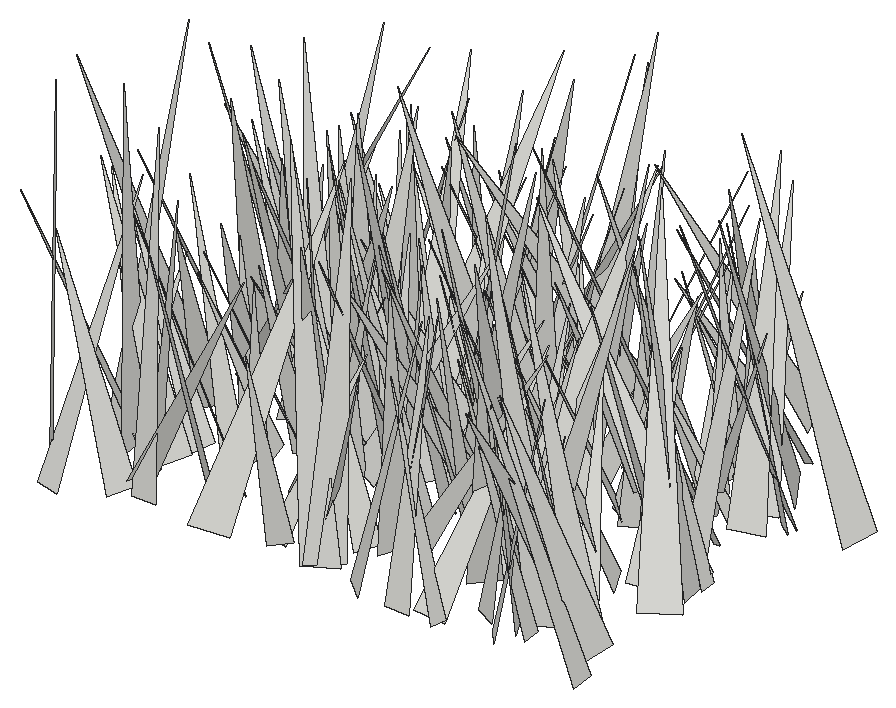
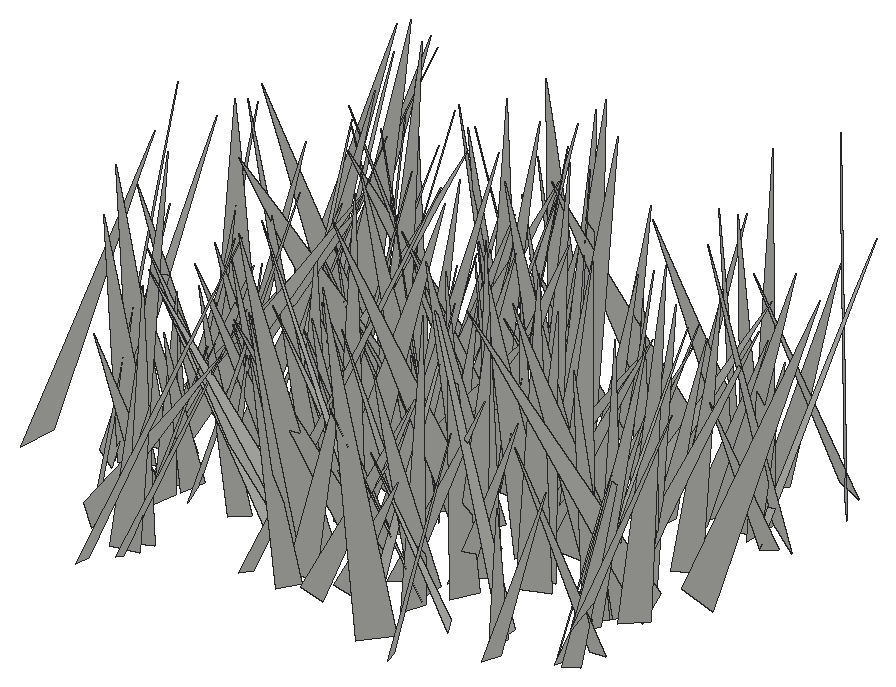
# SketchUp Ruby script. Lengths in inches.
U = 1.inch
M = Sketchup.active_model
def pt(a) = Geom::Point3d.new(a.map { |v| v * U })
def face(e, loops, mat)
  f = e.add_face(loops[0].map { |a| pt(a) })
  loops[1..].each { |l| e.add_face(l.map { |a| pt(a) }).erase! }
  f.material = f.back_material = mat if mat
  f
end
# faces: each face lists its corners as indices into pts; further lists are holes
def faces(e, pts, list, mat = nil) = list.each { |f| face(e, (f[0].is_a?(Array) ? f : [f]).map { |l| l.map { |i| pts[i] } }, mat) }
# xy, xz, yz: faces in a plane at the given z, y or x. An outline is a flat list of corners, or four numbers for a rectangle; further outlines are holes
def ring(l) = l.size == 4 ? [[l[0], l[1]], [l[2], l[1]], [l[2], l[3]], [l[0], l[3]]] : l.each_slice(2).to_a
def flat(e, list, mat, &to3) = list.each { |f| face(e, (f[0].is_a?(Array) ? f : [f]).map { |l| ring(l).map { |u, v| to3.(u, v) } }, mat) }
def xy(e, z, list, mat = nil) = flat(e, list, mat) { |x, y| [x, y, z] }
def xz(e, y, list, mat = nil) = flat(e, list, mat) { |x, z| [x, y, z] }
def yz(e, x, list, mat = nil) = flat(e, list, mat) { |y, z| [x, y, z] }
def lines(e, pts, list) = list.each { |a, b| e.add_line(pt(pts[a]), pt(pts[b])) }
# prism: a flat outline (further loops are holes) pulled along v
def prism(e, loops, v, mat = nil)
  f = face(e, loops, mat); d = Geom::Vector3d.new(v.map { |x| x * U })
  f.pushpull(f.normal.samedirection?(d) ? d.length : -d.length)
end
def box(e, o, s, mat = nil) = prism(e, [[o, [o[0] + s[0], o[1], o[2]], [o[0] + s[0], o[1] + s[1], o[2]], [o[0], o[1] + s[1], o[2]]]], [0, 0, s[2]], mat)
def at(x, y, z, deg = 0) = Geom::Transformation.translation(pt([x, y, z])) * Geom::Transformation.rotation(ORIGIN, Z_AXIS, deg.degrees)
def axes(o, x, y, z) = Geom::Transformation.new([*x, 0, *y, 0, *z, 0, *pt(o).to_a, 1])
def part(name) = M.definitions.add(name)
# library, detail: a bought-in or finely detailed component or shape, given as its bounding box
def library(name, o, s) = part(name).tap { |d| box(d.entities, o, s) }
def detail(e, o, s) = box(e.add_group.entities, o, s)
def put(e, d, t, mat = nil) = e.add_instance(d, t).tap { |i| i.material = mat if mat }
def group(e, t, mat = nil) = e.add_group.tap { |g| g.transformation = t; g.material = mat if mat }.entities
root = M.entities
c1 = part("fur_instance\#9")
p = [[0.8125,0,1.79],[0.67,-0.02,1.48],[0,-0.11,0],[0,0.11,0]]
faces(c1.entities,p,[[0,1,2,3]])
put(root,c1,axes([74.77,271.22,-27.1],[2.46831,-3.73303,1.12427],[-3.72872,-2.64901,-0.60947],[-1.13849,0.58247,4.43358]))
put(root,c1,axes([89.13,272.08,-27.1],[5.01755,-2.86523,2.69296],[-2.1597,-5.65647,-1.99435],[-3.28592,-0.6574,5.42291]))
put(root,c1,axes([90.02,270.07,-27.1],[-7.1325,-1.97369,0.04131],[-1.9512,7.0246,-1.27181],[-0.29997,1.23662,7.29044]))
put(root,c1,axes([67.68,270.7,-27.1],[-4.78062,2.36193,1.12593],[2.54726,4.73726,0.87783],[0.59826,-1.2963,5.25951]))
put(root,c1,axes([64.64,270.28,-27.1],[-5.7343,-4.84539,3.53032],[-5.45543,6.24306,-0.29262],[2.4858,2.5238,7.50162]))
put(root,c1,axes([71.45,271.63,-27.1],[-3.14093,-4.54056,1.19879],[-4.68857,3.11384,-0.49041],[0.26658,1.26749,5.49924]))
put(root,c1,axes([83.08,270.24,-27.1],[-4.76571,-0.2474,0.30777],[-0.30187,4.68534,-0.90794],[0.25457,0.92426,4.68496]))
put(root,c1,axes([86.31,274.4,-27.1],[4.64507,-4.79979,0.2726],[-4.36308,-4.36804,-2.56373],[-2.01887,-1.6035,6.16782]))
put(root,c1,axes([76.08,272.24,-27.1],[5.21952,0.68023,0.61562],[0.83808,-4.98198,-1.60081],[-0.37326,-1.674,5.01433]))
put(root,c1,axes([79.03,270.31,-27.1],[3.65147,4.43575,1.22236],[4.5601,-3.69672,-0.20725],[-0.61278,-1.07778,5.74161]))
put(root,c1,axes([81.28,270,-27.1],[0.82489,5.68831,1.342],[5.81529,-0.93413,0.38496],[-0.58339,-1.2684,5.73491]))
put(root,c1,axes([85.58,271.84,-27.1],[3.95748,1.9361,2.48086],[2.44941,-4.39763,-0.47534],[-1.97573,-1.57388,4.37997]))
put(root,c1,axes([84.11,271.7,-27.1],[-0.58036,-3.55618,1.37675],[-3.59236,0.97706,1.00942],[1.27936,1.13031,3.45894]))
put(root,c1,axes([85.32,270.69,-27.1],[3.56693,3.32971,1.1246],[3.34181,-3.70943,0.38354],[-1.08812,-0.47732,4.86445]))
put(root,c1,axes([67.83,271.52,-27.1],[5.28703,-2.12696,0.17156],[-2.11759,-5.17319,1.12251],[0.26309,1.10465,5.58719]))
put(root,c1,axes([79.96,271.45,-27.1],[5.42096,2.25752,1.64956],[2.38588,-5.61122,-0.16143],[-1.45775,-0.7887,5.87002]))
put(root,c1,axes([65.36,269.17,-27.1],[2.05142,5.93925,0.09208],[5.90467,-2.04959,0.65232],[-0.64654,0.12643,6.2496]))
put(root,c1,axes([86.4,271.58,-27.1],[-5.31837,-1.43549,0.4315],[-1.49067,5.23198,-0.96754],[0.15722,1.04767,5.42306]))
put(root,c1,axes([65.6,274.26,-27.1],[-4.61159,-4.4726,0.38091],[-4.39573,4.61032,0.9157],[0.90928,-0.396,6.35865]))
put(root,c1,axes([77.02,271.06,-27.1],[-5.99811,4.4385,2.51735],[4.45899,6.44808,-0.74453],[2.48087,-0.8583,7.4245]))
put(root,c1,axes([77.01,270.8,-27.1],[-1.50956,7.97784,1.83345],[8.07703,1.14872,1.65178],[-1.3301,-2.07864,7.94961]))
put(root,c1,axes([82.47,273.74,-27.1],[4.37125,-4.19897,0.80164],[-4.19734,-4.43318,-0.33332],[-0.81017,0.31203,6.05212]))
put(root,c1,axes([78.4,273.55,-27.1],[5.51508,-3.1001,1.56666],[-3.03836,-5.73026,-0.64316],[-1.68328,0.18611,6.29389]))
put(root,c1,axes([68.75,270.68,-27.1],[1.63726,6.8228,1.57078],[6.72877,-1.9791,1.58281],[-1.9343,-1.10957,6.83563]))
put(root,c1,axes([74.47,271.41,-27.1],[0.4921,4.23207,0.57816],[4.10963,-0.31046,-1.22532],[1.16432,-0.69285,4.08059]))
put(root,c1,axes([82.51,270.41,-27.1],[-2.22642,5.28944,0.76409],[4.89566,2.35054,-2.00661],[2.14349,0.12554,5.37668]))
put(root,c1,axes([67.1,273.39,-27.1],[3.49606,4.56093,2.47636],[5.16488,-3.35013,-1.12142],[-0.50841,-2.67048,5.63622]))
put(root,c1,axes([86.95,273.62,-27.1],[-5.18557,-4.32883,1.54546],[-4.49087,5.26797,-0.31293],[0.97941,1.23577,6.74766]))
put(root,c1,axes([86.36,272.54,-27.1],[-0.9931,7.68396,2.84346],[8.04191,0.36629,1.81887],[-1.56723,-2.98953,7.53135]))
put(root,c1,axes([77.51,273,-27.1],[-4.02277,2.62654,1.01722],[2.78428,3.97624,0.74391],[0.42575,-1.18612,4.74637]))
put(root,c1,axes([65.93,273.72,-27.1],[7.3985,0.06507,3.2704],[0.28828,-8.06925,-0.49163],[-3.25831,-0.56619,7.38244]))
put(root,c1,axes([72.08,270.36,-27.1],[-4.61251,5.93847,1.25396],[5.3205,4.71401,-2.75381],[2.92064,0.79104,6.99694]))
put(root,c1,axes([72.86,276.41,-27.1],[5.93446,-4.51627,0.11992],[-4.41947,-5.84426,-1.3935],[-0.93776,-1.03771,7.32616]))
put(root,c1,axes([71.45,273.29,-27.1],[-4.82792,-3.85999,0.34861],[-3.62589,4.30173,-2.58417],[-1.36894,2.21934,5.6152]))
put(root,c1,axes([67.8,273.71,-27.1],[-5.5849,2.54638,0.93821],[2.66389,5.55377,0.78405],[0.51763,-1.10771,6.08773]))
put(root,c1,axes([78.87,274.4375,-27.1],[4.45492,4.83666,0.95124],[4.56601,-3.56591,-3.25273],[1.85733,-2.83468,5.71483]))
put(root,c1,axes([87.88,273.12,-27.1],[-6.93734,1.12272,0.61983],[1.08478,6.95591,-0.45824],[0.68406,0.3553,7.01265]))
put(root,c1,axes([84.2,273.8125,-27.1],[-6.46812,-3.13785,1.21731],[-3.3431,6.29489,-1.53709],[0.38946,1.92167,7.02282]))
put(root,c1,axes([76.34,277.4,-27.1],[-2.99336,-6.46525,0.18966],[-6.30073,2.9619,1.52434],[1.46161,-0.47255,6.9596]))
put(root,c1,axes([74.34,274.375,-27.1],[-5.53367,-3.1899,2.46645],[-3.58117,5.81278,-0.51687],[1.85312,1.70777,6.3663]))
put(root,c1,axes([80.82,275.21,-27.1],[-3.26871,-2.2439,0.63682],[-2.29753,3.28654,-0.21245],[0.40248,0.53729,3.95909]))
put(root,c1,axes([74.2,274.79,-27.1],[-1.49797,-4.88201,2.75569],[-5.27998,2.18724,1.00478],[1.88406,2.24805,5.00683]))
put(root,c1,axes([70.18,275.58,-27.1],[3.44775,-2.42349,1.09947],[-2.43313,-3.5995,-0.30427],[-1.07797,0.37336,4.2033]))
put(root,c1,axes([80.49,275.58,-27.1],[-1.33118,-5.02308,1.66852],[-5.29255,1.28443,-0.35575],[0.06525,1.70478,5.18429]))
put(root,c1,axes([80.43,277.85,-27.1],[7.22069,-3.00234,1.05262],[-2.62839,-7.10035,-2.22196],[-1.79266,-1.6827,7.49769]))
put(root,c1,axes([86.3,276.83,-27.1],[-5.06216,-2.56794,0.53616],[-2.44101,5.03776,1.08155],[0.96086,-0.73072,5.57226]))
put(root,c1,axes([83.34,275.73,-27.1],[3.34183,1.38887,0.77255],[1.56239,-3.2005,-1.00466],[-0.29109,-1.23347,3.4767]))
put(root,c1,axes([67.99,275.08,-27.1],[-4.93751,1.50851,0.32737],[1.53378,4.91815,0.47027],[0.1741,-0.54591,5.14135]))
put(root,c1,axes([66.37,274.11,-27.1],[-3.43494,4.07646,0.13435],[4.04677,3.38429,0.77755],[-0.50915,-0.60283,5.27368]))
put(root,c1,axes([70.38,276.59,-27.1],[-4.26767,-0.91045,0.71231],[-0.70932,4.21373,1.13607],[0.91278,-0.98229,4.21323]))
put(root,c1,axes([79.55,277.92,-27.1],[1.60402,-6.13136,0.73735],[-5.58582,-1.76536,-2.52831],[-2.63361,0.00991,5.81155]))
put(root,c1,axes([78.98,274.86,-27.1],[-7.05105,-1.29004,0.36767],[-1.33665,6.92247,-1.34515],[0.11284,1.38992,7.04075]))
put(root,c1,axes([64.91,274.48,-27.1],[-0.81178,3.59213,0.55552],[3.51446,0.92094,-0.81938],[0.92765,-0.34562,3.5904]))
put(root,c1,axes([84.94,276,-27.1],[-4.9499,-5.12629,0.49866],[-4.98162,4.58947,-2.26921],[-1.30806,1.92014,6.75508]))
put(root,c1,axes([84.68,273.64,-27.1],[6.67924,-1.26552,2.75336],[-2.18749,-6.62541,2.26131],[-2.097,2.88046,6.41095]))
put(root,c1,axes([71.25,277.23,-27.1],[1.69834,-4.62751,0.65795],[-4.61755,-1.76962,-0.52709],[-0.72459,0.43091,4.90106]))
put(root,c1,axes([66.21,277.76,-27.1],[3.84252,-3.67557,0.42443],[-3.56655,-3.84235,-0.9854],[-0.98471,-0.42605,5.2253]))
put(root,c1,axes([75.875,276.62,-27.1],[-6.16765,-3.82155,1.90605],[-3.98751,6.35208,-0.16723],[1.52874,1.15063,7.2537]))
put(root,c1,axes([81.23,276.02,-27.1],[-3.53133,-2.30027,1.49102],[-2.55807,3.63918,-0.44418],[0.98523,1.20406,4.19097]))
put(root,c1,axes([71.56,276.83,-27.1],[-3.04212,-3.44962,0.11938],[-3.35963,2.92271,-1.15727],[-0.79185,0.85236,4.45141]))
put(root,c1,axes([65.06,273.51,-27.1],[3.59561,7.30217,1.1805],[7.09033,-3.77639,1.76345],[-2.10771,-0.24675,7.94609]))
put(root,c1,axes([72.86,276.56,-27.1],[1.59006,-7.38899,3.46765],[-7.94346,-2.21328,-1.07372],[-1.87702,3.10714,7.48148]))
put(root,c1,axes([69.16,275.47,-27.1],[-5.26641,1.25593,0.32091],[1.22212,5.2582,-0.5227],[0.43216,0.43524,5.3888]))
put(root,c1,axes([86.23,275.01,-27.1],[-2.52047,3.62206,0.22803],[3.61381,2.53037,-0.24846],[0.33426,-0.04477,4.40572]))
put(root,c1,axes([72.46,274.8,-27.1],[4.05537,2.07279,0.17475],[1.9711,-3.95155,1.12829],[-0.66463,0.92835,4.41242]))
put(root,c1,axes([73.86,276.52,-27.1],[-6.94561,0.7265,2.56424],[0.79665,7.39636,0.06233],[2.54332,-0.33278,6.98322]))
put(root,c1,axes([82.72,274.9,-27.1],[1.79845,4.31058,0.12569],[4.2592,-1.79684,0.67963],[-0.67534,0.14702,4.621]))
put(root,c1,axes([78.66,278.54,-27.1],[-0.3519,-5.66898,0.64957],[-5.59847,0.21723,-1.13712],[-1.1029,0.70611,5.5649]))
put(root,c1,axes([76.5,276.26,-27.1],[2.39277,4.07076,1.54907],[4.21231,-2.6123,0.35825],[-1.10775,-1.14055,4.7083]))
put(root,c1,axes([74.09,277.85,-27.1],[-1.49578,-4.28811,0.26565],[-3.87905,1.22698,-2.03551],[-1.84701,0.89578,4.0598]))
put(root,c1,axes([82.9,281.16,-27.1],[-3.72735,-5.65721,0.3773],[-4.71825,3.34531,3.54775],[3.14396,-1.68653,5.77153]))
put(root,c1,axes([78.07,277.09,-27.1],[-2.85535,-4.62994,1.75531],[-4.89429,2.33192,-1.81068],[-0.75056,2.40755,5.12941]))
put(root,c1,axes([66.88,279.6,-27.1],[4.17409,-3.35782,0.27535],[-3.2273,-4.11088,-1.20788],[-0.96712,-0.77425,5.2191]))
put(root,c1,axes([75.68,279.16,-27.1],[0.67121,-5.58126,0.90748],[-5.6399,-0.72653,-0.2969],[-0.40679,0.86382,5.61363]))
put(root,c1,axes([74.67,279.74,-27.1],[-1.5232,-7.73744,1.34983],[-7.81047,1.63722,0.57115],[0.82858,1.20901,7.86523]))
put(root,c1,axes([67.85,278.87,-27.1],[-3.27123,-4.88451,0.3113],[-4.82797,3.15879,-1.17003],[-0.80376,0.90546,5.76111]))
put(root,c1,axes([70.71,278.64,-27.1],[5.42547,-4.53511,0.52895],[-4.56014,-5.3411,0.98008],[0.2284,1.09004,7.00303]))
put(root,c1,axes([81.42,280.06,-27.1],[-5.10979,-2.8974,1.28802],[-2.4355,5.15064,1.92434],[2.03034,-1.11347,5.54994]))
put(root,c1,axes([86.8,279.02,-27.1],[-2.84226,-5.05917,1.08036],[-5.16298,2.85167,-0.22901],[0.32566,1.05526,5.79838]))
put(root,c1,axes([81.97,276.77,-27.1],[0.88242,4.55252,0.64978],[4.54635,-0.76413,-0.82042],[0.6916,-0.78549,4.5641]))
put(root,c1,axes([73.89,277.25,-27.1],[1.55014,5.60518,1.20615],[5.3228,-0.94254,-2.46072],[2.13086,-1.72318,5.26933]))
put(root,c1,axes([76.1875,278.51,-27.1],[-3.70212,4.89762,1.86065],[5.19102,3.12087,2.11373],[-0.70854,-2.72541,5.76407]))
put(root,c1,axes([64.6,279.16,-27.1],[-0.79345,-6.87819,1.77521],[-6.83318,0.25089,-2.08208],[-1.94125,1.92821,6.60333]))
put(root,c1,axes([89.12,277.74,-27.1],[-6.73527,-1.87686,1.53677],[-2.12146,6.75676,-1.04577],[1.17629,1.43931,6.91323]))
put(root,c1,axes([89.02,275.93,-27.1],[-3.36629,7.35026,0.38103],[7.33966,3.3212,0.77612],[-0.54849,-0.66835,8.0471]))
put(root,c1,axes([67.26,278.79,-27.1],[1.04159,-3.44564,1.2731],[-3.64709,-1.12789,-0.06873],[-0.4381,1.19732,3.59897]))
put(root,c1,axes([75.13,277.36,-27.1],[-0.50295,4.78104,0.71911],[4.81704,0.43358,0.48636],[-0.41423,-0.76294,4.78276]))
put(root,c1,axes([89.18,278.61,-27.1],[-3.86057,-0.50737,0.50019],[-0.53854,3.88252,-0.21837],[0.46646,0.28336,3.88764]))
put(root,c1,axes([82.76,274.6,-27.1],[-6.00676,5.62271,0.83771],[4.81686,5.68135,-3.59416],[3.01902,2.12255,7.40122]))
put(root,c1,axes([87.07,277.01,-27.1],[0.03105,4.61747,0.04613],[4.59439,-0.03553,0.46309],[-0.46341,-0.04278,4.59429]))
put(root,c1,axes([77.5,280.37,-27.1],[3.26712,2.26093,2.86418],[3.20778,-3.61207,-0.80776],[-1.73938,-2.41465,3.89016]))
put(root,c1,axes([88.39,279.12,-27.1],[-2.47066,2.78913,0.64805],[2.82871,2.24449,1.12431],[-0.44456,-1.21919,3.55237]))
put(root,c1,axes([76.47,278.97,-27.1],[-0.19493,4.51759,1.73565],[4.75586,-0.14282,0.90585],[-0.89608,-1.74071,4.43013]))
put(root,c1,axes([78.51,280.02,-27.1],[-2.5232,4.5633,1.53247],[4.25008,1.29942,3.12842],[-2.26029,-2.65076,4.17172]))
put(root,c1,axes([76.4,278.7,-27.1],[1.55212,3.88569,0.28277],[3.69063,-1.36892,-1.44671],[1.24813,-0.78428,3.92616]))
put(root,c1,axes([77.59,278.71,-27.1],[6.54484,-1.1484,2.12677],[-1.53141,-6.71985,1.08414],[-1.86996,1.48383,6.55579]))
put(root,c1,axes([88.48,278.59,-27.1],[-3.77529,6.85051,0.02559],[5.94676,3.26269,3.89536],[-3.40091,-1.89957,6.78296]))
put(root,c1,axes([72.57,279.15,-27.1],[-0.09344,5.23116,1.72248],[5.50098,0.0052,0.28262],[-0.26677,-1.725,5.22436]))
put(root,c1,axes([76.12,280.08,-27.1],[6.04593,4.4435,2.18806],[4.86244,-5.98205,-1.28733],[-0.94282,-2.35709,7.39194]))
put(root,c1,axes([71.57,280.19,-27.1],[-3.32714,-4.87132,0.7615],[-4.7527,2.92423,-2.05917],[-1.31203,1.7603,5.52806]))
put(root,c1,axes([84.7,281.12,-27.1],[-1.00098,-5.50903,0.83943],[-5.47181,0.81017,-1.20786],[-1.05515,1.02481,5.46739]))
put(root,c1,axes([65.36,281.95,-27.1],[6.33398,-2.31725,1.64534],[-1.9481,-6.46653,-1.60778],[-2.06922,-1.00519,6.55011]))
put(root,c1,axes([66.53,282.64,-27.1],[6.05103,1.03829,2.78411],[2.19851,-5.8136,-2.61017],[-1.99898,-3.2509,5.55698]))
put(root,c1,axes([80.48,278.93,-27.1],[0.12612,4.07155,0.3622],[4.08216,-0.1442,0.19951],[-0.2114,-0.35539,4.06861]))
put(root,c1,axes([82.58,279.52,-27.1],[-4.08375,3.22336,1.0157],[3.24667,4.18417,-0.22495],[0.93853,-0.4488,5.19774]))
put(root,c1,axes([70.18,279.49,-27.1],[-1.69454,7.12423,1.83382],[7.32335,1.45532,1.11334],[-0.69716,-2.02889,7.23786]))
put(root,c1,axes([76.58,282.52,-27.1],[-7.9399,0.37328,2.34081],[0.92834,8.01881,1.87016],[2.18103,-2.05426,7.72553]))
put(root,c1,axes([71.34,280.36,-27.1],[-3.27295,5.40819,2.7555],[5.57889,3.91368,-1.05481],[2.39109,-1.7286,6.23283]))
put(root,c1,axes([81.21,281.02,-27.1],[-2.12698,-6.60371,3.80122],[-7.1046,3.14508,1.48842],[2.75369,3.0136,6.77625]))
put(root,c1,axes([66.2,282.33,-27.1],[5.00192,-1.81934,1.03799],[-1.65,-5.07776,-0.94895],[-1.29032,-0.55947,5.23724]))
put(root,c1,axes([76.47,279.89,-27.1],[-1.50833,4.20798,0.27956],[4.21722,1.50618,0.08227],[0.01672,-0.29093,4.46939]))
put(root,c1,axes([70.14,281.59,-27.1],[1.65081,-5.08845,2.41171],[-5.51574,-1.96719,-0.37505],[-1.13372,2.16141,5.33637]))
put(root,c1,axes([87.43,281.31,-27.1],[-5.76145,-5.93812,0.42997],[-5.44241,5.01036,-3.73055],[-2.41379,2.87671,7.38502]))
put(root,c1,axes([67.625,281.76,-27.1],[-5.88104,-3.53705,0.94417],[-3.64814,5.81133,-0.9531],[0.30541,1.30636,6.79625]))
put(root,c1,axes([78.9375,281.93,-27.1],[-0.03383,-6.90938,2.82252],[-7.12958,-0.80509,-2.05628],[-2.20801,2.70547,6.5964]))
put(root,c1,axes([69.74,282.43,-27.1],[2.04038,-5.82637,1.87095],[-6.1057,-2.07021,0.21174],[-0.4092,1.83789,6.16967]))
put(root,c1,axes([87.95,279.14,-27.1],[1.53889,6.65129,0.3221],[6.53467,-1.57198,1.24039],[-1.28121,-0.02868,6.71336]))
put(root,c1,axes([83.02,280.94,-27.1],[1.48501,3.27806,0.44782],[3.28348,-1.52047,0.24164],[-0.40618,-0.30651,3.59062]))
put(root,c1,axes([69.33,278.88,-27.1],[-6.96616,2.88196,1.8212],[2.05018,6.85162,-3.00033],[2.72382,2.21349,6.91601]))
put(root,c1,axes([66.6,282.59,-27.1],[2.66304,-4.00114,1.09323],[-4.14622,-2.60379,0.57024],[-0.11461,1.22768,4.77239]))
put(root,c1,axes([71.75,282.63,-27.1],[-0.58668,-6.43534,2.37936],[-6.81319,0.82822,0.56013],[0.80964,2.30643,6.43771]))
put(root,c1,axes([67.8,281.625,-27.1],[-4.98087,1.16288,0.32288],[1.15979,4.99131,-0.08543],[0.33384,0.00996,5.1141]))
put(root,c1,axes([78.16,282.82,-27.1],[0.12589,-6.48138,2.39431],[-6.90548,-0.03647,0.26437],[0.23531,2.39734,6.47721]))
put(root,c1,axes([86.71,283.21,-27.1],[-3.57731,-0.93265,0.01118],[-0.92223,3.54345,0.51048],[0.1395,-0.49118,3.66148]))
put(root,c1,axes([88.41,284.49,-27.1],[-4.17901,-5.88434,0.7845],[-5.89024,4.22956,0.34775],[0.73891,0.43633,7.20893]))
put(root,c1,axes([74.07,279.99,-27.1],[-5.45003,5.37343,0.92209],[5.18096,5.51046,-1.48977],[1.69756,0.43353,7.50714]))
put(root,c1,axes([85.92,282.64,-27.1],[4.29201,-0.29938,0.77765],[-0.39482,-4.32378,0.51456],[-0.73381,0.57535,4.27156]))
put(root,c1,axes([83.32,283.51,-27.1],[-4.36965,-1.59831,1.51111],[-1.58231,4.61869,0.30967],[1.52785,0.21216,4.64247]))
put(root,c1,axes([80.67,282.76,-27.1],[0.36945,4.73641,1.83647],[4.53767,0.52011,-2.25427],[2.28381,-1.79961,4.18191]))
put(root,c1,axes([66.42,283.5,-27.1],[-6.02827,1.48886,1.73676],[1.72693,6.17226,0.7029],[1.50026,-1.12234,6.1695]))
put(root,c1,axes([72.23,283.13,-27.1],[-4.31803,3.62073,2.04082],[3.93255,4.51165,0.31626],[1.34522,-1.56695,5.62628]))
put(root,c1,axes([71.5,284.3,-27.1],[5.97247,-1.71505,1.0533],[-1.60325,-6.04797,-0.7569],[-1.21673,-0.44932,6.16757]))
put(root,c1,axes([65.51,280.73,-27.1],[7.33228,1.89466,0.16833],[1.78282,-7.07911,2.02191],[-0.66303,1.91751,7.29821]))
put(root,c1,axes([77.83,283.27,-27.1],[-3.1989,2.68909,0.37978],[2.66785,3.00183,1.21655],[-0.50792,-1.16886,3.99802]))
put(root,c1,axes([87.21,286.36,-27.1],[-6.01376,-4.74049,2.00405],[-3.98095,6.23797,2.80955],[3.26197,-1.12665,7.12348]))
put(root,c1,axes([84.18,284.57,-27.1],[-6.24569,-2.79636,0.92417],[-2.76847,6.31368,0.39421],[1.00464,0.01396,6.83176]))
put(root,c1,axes([84.02,280.32,-27.1],[2.20032,6.76237,0.49836],[6.15454,-2.21163,2.83722],[-2.84601,0.44546,6.52083]))
put(root,c1,axes([73.3,281.09,-27.1],[-0.97355,8.05143,1.14446],[7.84551,1.23329,-2.00251],[2.14086,-0.85824,7.85896]))
put(root,c1,axes([72.33,283.625,-27.1],[-3.83694,1.86592,0.39498],[1.90547,3.78872,0.61201],[0.08273,-0.72368,4.22246]))
put(root,c1,axes([78.17,281.66,-27.1],[4.5765,3.32185,0.66717],[3.07667,-4.544,1.52],[-1.41913,0.86116,5.4469]))
put(root,c1,axes([79,287.91,-27.1],[-7.67561,-3.02253,0.64542],[-2.50236,7.09168,3.4516],[1.81396,-3.00659,7.49247]))
put(root,c1,axes([88.69,283.76,-27.1],[2.96491,4.33641,3.25393],[4.46173,-4.05854,1.34327],[-3.07985,-1.70497,5.07846]))
put(root,c1,axes([75.94,284.24,-27.1],[3.19259,1.80159,0.09548],[1.75198,-3.04965,-1.03811],[0.43061,-0.9494,3.51578]))
put(root,c1,axes([65.07,286.03,-27.1],[-4.32761,-0.50237,2.11035],[0.41917,4.42689,1.9134],[2.12844,-1.89326,3.91401]))
put(root,c1,axes([65.59,285.91,-27.1],[-5.22696,-1.19875,0.73288],[-0.94186,5.08442,1.59898],[1.04259,-1.41663,5.11873]))
put(root,c1,axes([85.04,284.3125,-27.1],[-2.3678,2.48019,1.72309],[2.76192,2.66404,-0.03926],[1.22155,-1.2159,3.42875]))
put(root,c1,axes([81.79,284.79,-27.1],[1.56073,-4.1385,0.9971],[-4.17951,-1.28812,1.1957],[0.80812,1.33073,4.25833]))
put(root,c1,axes([75.71,283.56,-27.1],[4.89085,0.64493,0.58721],[0.56841,-4.89366,0.64042],[-0.66156,0.56328,4.89144]))
put(root,c1,axes([77.01,283.89,-27.1],[-2.42701,4.03219,1.90827],[4.11447,2.86278,-0.81615],[1.72373,-1.15601,4.63496]))
put(root,c1,axes([65.98,285.68,-27.1],[-3.08221,-2.2445,0.63722],[-2.14243,3.14072,0.69983],[0.92405,-0.20483,3.74807]))
put(root,c1,axes([87.73,282.71,-27.1],[-1.40207,7.22786,1.13046],[7.31414,1.36087,0.37039],[-0.15287,-1.17973,7.35327]))
put(root,c1,axes([74.11,284.93,-27.1],[-4.51711,1.79985,0.33219],[1.82954,4.41557,0.95372],[-0.05124,-1.00862,4.76803]))
put(root,c1,axes([74.78,283.1,-27.1],[4.77639,3.07128,1.21309],[2.81816,-4.90311,1.31748],[-1.72115,0.49496,5.52367]))
put(root,c1,axes([68.45,285.57,-27.1],[6.75177,1.95337,0.7466],[2.07523,-6.56983,-1.57805],[-0.25785,-1.72661,6.84922]))
put(root,c1,axes([91.35,284.875,-27.1],[-8.2127,0.65784,0.53458],[0.66874,8.22786,0.14871],[0.52088,-0.19122,8.23766]))
put(root,c1,axes([85.98,284.9,-27.1],[-4.15206,-1.52587,0.16301],[-1.50616,3.96212,-1.27574],[-0.29385,1.25209,4.2356]))
put(root,c1,axes([72.42,286.21,-27.1],[5.48977,-0.87036,1.92832],[-0.64898,-5.79667,-0.76876],[-2.01365,-0.50463,5.50492]))
put(root,c1,axes([80.62,284.52,-27.1],[4.47916,2.33614,0.04477],[2.33654,-4.47877,-0.05982],[-0.01203,-0.07375,5.05142]))
put(root,c1,axes([72.76,288.58,-27.1],[-3.43989,-5.36661,0.1848],[-4.97328,3.26677,2.29397],[2.02515,-1.09328,5.94736]))
put(root,c1,axes([80.82,284.24,-27.1],[5.67742,2.27779,0.25934],[2.25803,-5.67581,0.41845],[-0.39608,0.29237,6.10297]))
put(root,c1,axes([64.92,284.66,-27.1],[1.35315,4.35582,0.79538],[4.34518,-1.14634,-1.11449],[0.85157,-1.07217,4.42291]))
put(root,c1,axes([84.51,284.2,-27.1],[-3.56654,2.39752,0.7344],[2.22273,3.6139,-1.00345],[1.16058,0.44646,4.17868]))
put(root,c1,axes([87.25,284.09,-27.1],[-2.49742,5.95651,1.04282],[6.02179,2.55284,-0.16018],[0.55273,-0.89868,6.45689]))
put(root,c1,axes([84.79,285.55,-27.1],[-4.53937,1.16522,1.40638],[1.15678,4.75002,-0.2018],[1.41333,-0.14527,4.6822]))
put(root,c1,axes([75.87,284.27,-27.1],[6.07013,4.91373,1.22638],[4.90353,-6.18107,0.495],[-1.26656,-0.38061,7.79399]))
put(root,c1,axes([79.71,284.1,-27.1],[5.6659,3.07924,0.02777],[3.03508,-5.59401,1.03936],[-0.52039,0.90013,6.36426]))
put(root,c1,axes([75.3,284.76,-27.1],[5.97099,-0.01983,0.33196],[-0.11666,-5.7151,1.75709],[-0.31141,1.76085,5.70664]))
put(root,c1,axes([83.57,289.4,-27.1],[-0.94018,-7.50089,0.47804],[-7.29693,1.02641,1.75419],[1.80188,0.24278,7.35324]))
put(root,c1,axes([76.66,286.9,-27.1],[-2.71564,-2.49022,0.0198],[-2.39499,2.6036,-1.03032],[-0.68234,0.77224,3.53756]))
put(root,c1,axes([72.93,285.23,-27.1],[2.99625,3.60782,0.19235],[3.59342,-3.00177,0.328],[-0.37513,0.06212,4.67828]))
put(root,c1,axes([76.03,287.73,-27.1],[0.12283,-4.44104,1.09952],[-4.1986,-0.54638,-1.73783],[-1.81756,0.96203,4.08875]))
put(root,c1,axes([72.66,285.12,-27.1],[4.91626,-1.03874,2.91243],[-2.03601,-5.20453,1.58061],[-2.3272,2.35896,4.76972]))
put(root,c1,axes([83.875,288.38,-27.1],[-3.49973,-1.74713,0.54329],[-1.50598,3.41664,1.28623],[1.03907,-0.93268,3.69408]))
put(root,c1,axes([85.03,285.88,-27.1],[3.51726,-1.23078,1.44078],[-1.67757,-3.4351,1.16087],[-0.88116,1.62697,3.54095]))
put(root,c1,axes([77.2,286.87,-27.1],[1.69917,-3.99461,2.49122],[-4.30676,-2.38859,-0.89256],[-1.90128,1.84064,4.24822]))
put(root,c1,axes([77.07,287.77,-27.1],[3.70766,-2.56946,0.56874],[-2.62102,-3.69364,0.39947],[-0.23628,0.65362,4.49325]))
put(root,c1,axes([67.79,287.38,-27.1],[-4.13289,0.76106,0.51137],[0.79822,4.14817,0.27763],[0.45116,-0.36746,4.1932]))
put(root,c1,axes([70.53,286.44,-27.1],[3.48298,2.03603,0.22687],[2.02285,-3.48877,0.25421],[-0.32396,0.10555,4.02641]))
put(root,c1,axes([77.51,285.6,-27.1],[-6.57541,3.25527,2.97746],[2.73361,7.20101,-1.83599],[3.46258,0.49673,7.10365]))
put(root,c1,axes([68.23,286.42,-27.1],[-3.61922,1.27993,0.57976],[1.16278,3.62754,-0.74965],[0.78884,0.52519,3.76496]))
put(root,c1,axes([83.35,288.72,-27.1],[1.74282,-4.6233,0.69197],[-4.67126,-1.6936,0.44965],[0.18179,0.80496,4.92038]))
put(root,c1,axes([75.23,286.8,-27.1],[-1.27036,4.00789,0.19304],[3.62684,1.0603,1.85365],[-1.71652,-0.72583,3.77372]))
put(root,c1,axes([86.24,288.26,-27.1],[-2.89235,-4.23355,0.19447],[-3.82387,2.50545,-2.32964],[-1.82723,1.45817,4.56743]))
put(root,c1,axes([83.37,289.95,-27.1],[-4.08154,-1.42978,0.42723],[-1.12455,3.76494,1.85644],[0.98091,-1.633,3.906]))
put(root,c1,axes([72.06,288.85,-27.1],[4.17452,-5.37379,1.20818],[-5.50555,-4.02647,1.11376],[0.16212,1.6352,6.71296]))
put(root,c1,axes([84.24,291.08,-27.1],[-6.53247,-2.60599,0.49941],[-2.30056,6.22381,2.3844],[1.32211,-2.04617,6.61657]))
put(root,c1,axes([78.19,286.14,-27.1],[2.36714,6.37429,1.14743],[6.22522,-2.57637,1.46983],[-1.78738,-0.5313,6.63886]))
put(root,c1,axes([70.78,289.6,-27.1],[-3.9819,-2.09854,0.99873],[-1.89028,4.07705,1.03024],[1.35209,-0.4803,4.38155]))
